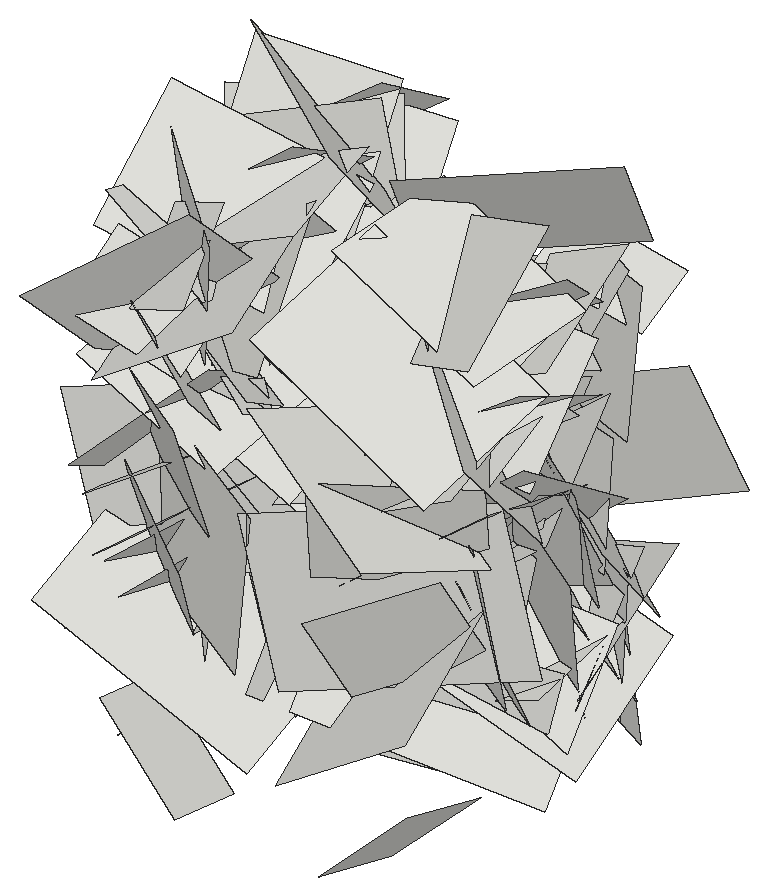
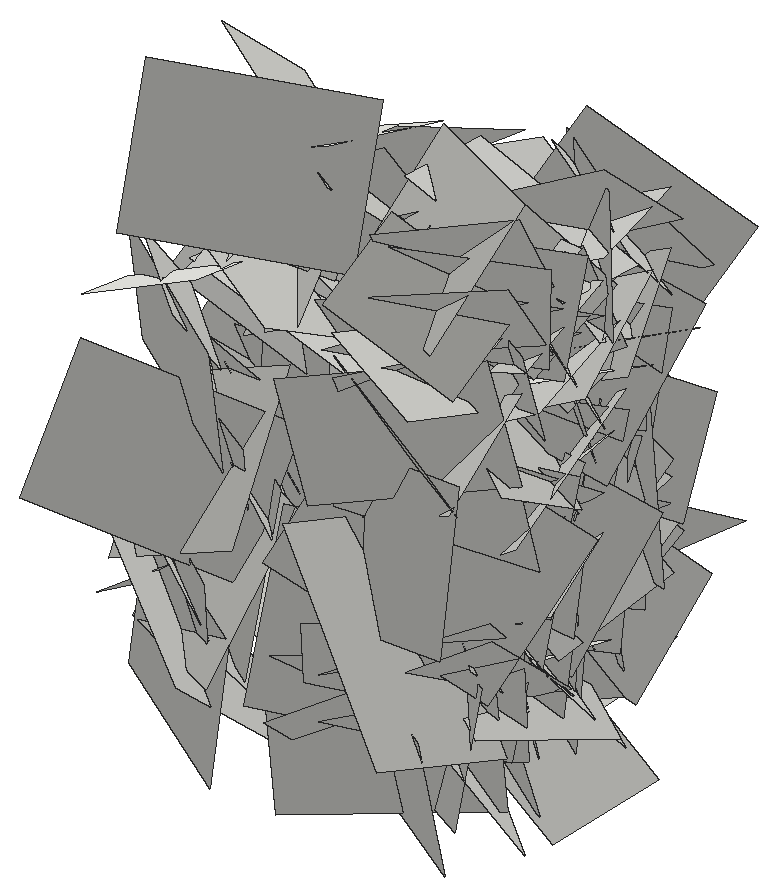
# SketchUp Ruby script. Lengths in inches.
U = 1.inch
M = Sketchup.active_model
def pt(a) = Geom::Point3d.new(a.map { |v| v * U })
def face(e, loops, mat)
  f = e.add_face(loops[0].map { |a| pt(a) })
  loops[1..].each { |l| e.add_face(l.map { |a| pt(a) }).erase! }
  f.material = f.back_material = mat if mat
  f
end
# faces: each face lists its corners as indices into pts; further lists are holes
def faces(e, pts, list, mat = nil) = list.each { |f| face(e, (f[0].is_a?(Array) ? f : [f]).map { |l| l.map { |i| pts[i] } }, mat) }
# xy, xz, yz: faces in a plane at the given z, y or x. An outline is a flat list of corners, or four numbers for a rectangle; further outlines are holes
def ring(l) = l.size == 4 ? [[l[0], l[1]], [l[2], l[1]], [l[2], l[3]], [l[0], l[3]]] : l.each_slice(2).to_a
def flat(e, list, mat, &to3) = list.each { |f| face(e, (f[0].is_a?(Array) ? f : [f]).map { |l| ring(l).map { |u, v| to3.(u, v) } }, mat) }
def xy(e, z, list, mat = nil) = flat(e, list, mat) { |x, y| [x, y, z] }
def xz(e, y, list, mat = nil) = flat(e, list, mat) { |x, z| [x, y, z] }
def yz(e, x, list, mat = nil) = flat(e, list, mat) { |y, z| [x, y, z] }
def lines(e, pts, list) = list.each { |a, b| e.add_line(pt(pts[a]), pt(pts[b])) }
# prism: a flat outline (further loops are holes) pulled along v
def prism(e, loops, v, mat = nil)
  f = face(e, loops, mat); d = Geom::Vector3d.new(v.map { |x| x * U })
  f.pushpull(f.normal.samedirection?(d) ? d.length : -d.length)
end
def box(e, o, s, mat = nil) = prism(e, [[o, [o[0] + s[0], o[1], o[2]], [o[0] + s[0], o[1] + s[1], o[2]], [o[0], o[1] + s[1], o[2]]]], [0, 0, s[2]], mat)
def at(x, y, z, deg = 0) = Geom::Transformation.translation(pt([x, y, z])) * Geom::Transformation.rotation(ORIGIN, Z_AXIS, deg.degrees)
def axes(o, x, y, z) = Geom::Transformation.new([*x, 0, *y, 0, *z, 0, *pt(o).to_a, 1])
def part(name) = M.definitions.add(name)
# library, detail: a bought-in or finely detailed component or shape, given as its bounding box
def library(name, o, s) = part(name).tap { |d| box(d.entities, o, s) }
def detail(e, o, s) = box(e.add_group.entities, o, s)
def put(e, d, t, mat = nil) = e.add_instance(d, t).tap { |i| i.material = mat if mat }
def group(e, t, mat = nil) = e.add_group.tap { |g| g.transformation = t; g.material = mat if mat }.entities
root = M.entities
c1 = part("Component\#6")
p = [[0.01,0,0],[0,3.24,4.54],[4.32,3.24,4.54],[4.33,0,0]]
faces(c1.entities,p,[[0,1,2,3]])
put(root,c1,axes([410.71,199.18,25.47],[0.11604,-0.3767,0.6399],[-0.02749,0.64448,0.38383],[0.78661,0.07809,-0.08099]))
put(root,c1,axes([410.71,201.02,32],[-0.03236,-0.79816,-0.43551],[-0.07074,-0.43262,0.79753],[0.9612,-0.0587,0.04403]))
put(root,c1,axes([414.68,202.06,39.63],[0.00244,-0.36914,-0.6705],[-0.07457,-0.66776,0.36739],[-0.80789,0.06052,-0.03594]))
put(root,c1,axes([410.71,194.18,31.13],[-0.04063,-0.16003,0.87853],[-0.02386,0.87924,0.15917],[0.94627,0.0153,0.04174]))
put(root,c1,axes([410.71,191.375,35.34],[0.1473,0.40574,0.51918],[0.07991,0.51733,-0.42447],[0.69387,-0.14571,-0.06134]))
put(root,c1,axes([414.68,192.92,34.17],[0.15147,-0.1521,1.01718],[0.1212,1.02293,0.1369],[-1.08344,0.09316,0.15752]))
put(root,c1,axes([414.68,201.02,39.48],[0.13577,0.09163,-0.9618],[0.05798,-0.96935,-0.08506],[-1.02248,-0.0428,-0.13253]))
put(root,c1,axes([414.68,193.07,33.95],[-0.05953,0.85388,-0.40475],[0.24794,-0.38029,-0.83472],[-0.97048,-0.14953,-0.18843]))
put(root,c1,axes([410.71,198.86,35.2],[-0.14047,0.16017,0.87964],[0.13868,0.88315,-0.1411],[0.93754,-0.10664,0.15267]))
put(root,c1,axes([410.71,198.41,25.5],[-0.14641,-1.02966,0.26735],[-0.10928,0.28128,1.03005],[1.12233,-0.10694,0.13517]))
put(root,c1,axes([414.68,192.38,31.46],[-0.05244,0.73173,-0.11131],[-0.01157,-0.11227,-0.73318],[-0.78447,-0.04726,0.01825]))
put(root,c1,axes([414.68,195.89,35.57],[0.03273,-0.74668,0.19464],[-0.06894,0.19158,0.74527],[-0.81502,-0.04619,-0.05522]))
put(root,c1,axes([410.71,195.33,34.42],[0.12228,0.30682,0.85432],[-0.19875,0.85067,-0.2802],[0.94146,0.13973,-0.17012]))
put(root,c1,axes([410.71,197.53,26.62],[0.11622,-0.11144,-0.6986],[0.08861,-0.69994,0.12478],[0.74462,0.10068,0.09418]))
put(root,c1,axes([414.68,194.17,31.15],[0.1572,-0.65225,0.62778],[0.00257,0.63643,0.66066],[-0.9596,-0.10514,0.10461]))
put(root,c1,axes([414.68,196.95,39.61],[0.06663,0.78722,-0.39485],[0.0883,-0.3994,-0.78302],[-0.92935,0.01849,-0.10271]))
put(root,c1,axes([410.71,195.16,37.28],[0.08536,-0.54597,-0.55526],[0.06407,-0.55215,0.55168],[0.82294,0.09962,0.01464]))
put(root,c1,axes([410.71,201.91,26.14],[-0.02369,0.31708,-0.9382],[-0.09459,-0.93526,-0.31396],[1.04548,-0.07743,-0.04967]))
put(root,c1,axes([414.68,198.57,33.25],[0.09717,0.14422,-0.89801],[0.11089,-0.89824,-0.13357],[-0.95769,-0.08937,-0.10658]))
put(root,c1,axes([410.71,200.1,34.99],[0.01875,0.74709,-0.59948],[-0.09315,-0.59579,-0.74508],[1.01106,-0.06874,-0.05753]))
put(root,c1,axes([414.68,192.15,39.48],[0.21361,0.71392,-0.72381],[0.12034,-0.74908,-0.70723],[-1.07091,0.05823,-0.22384]))
put(root,c1,axes([410.71,204.82,25.65],[-0.12938,-0.11687,-1.00907],[0.02351,-1.01639,0.11504],[1.07651,0.00815,-0.12379]))
put(root,c1,axes([414.68,197.17,21.41],[0.31691,0.51794,0.91951],[0.05422,0.94746,-0.55031],[-1.11735,0.19287,0.23409]))
put(root,c1,axes([410.71,195.4,26.27],[0.15303,-0.80886,0.21466],[-0.08059,0.20425,0.82078],[0.8834,0.15875,0.0377]))
put(root,c1,axes([410.71,195.7,29.31],[-0.12944,0.87645,-0.3909],[0.13192,-0.37627,-0.88251],[1.00866,0.16168,0.06525]))
put(root,c1,axes([414.68,199.74,34.07],[-0.11183,-0.60219,-0.2199],[0.02555,-0.22643,0.6085],[-0.67907,0.09065,0.0591]))
put(root,c1,axes([414.68,201.07,39.9375],[0.03161,0.68058,-0.41337],[0.06223,-0.41441,-0.67806],[-0.84176,-0.00508,-0.06565]))
put(root,c1,axes([410.71,195.45,23.05],[0.08121,0.42866,0.62692],[0.16296,0.6083,-0.43472],[0.78836,-0.1699,0.02528]))
put(root,c1,axes([414.68,196.5,26.6],[0.00001,0.64808,0.59207],[0.20568,0.57742,-0.63205],[-0.90746,0.13088,-0.14325]))
put(root,c1,axes([410.71,200.17,25.9],[0.12286,-0.34825,-0.84521],[-0.12526,-0.85054,0.33424],[0.96086,-0.06635,0.15165]))
put(root,c1,axes([410.71,194.92,22.54],[0.07164,-0.895,0.57486],[-0.24411,0.55005,0.88344],[1.1008,0.18023,0.15849]))
put(root,c1,axes([410.71,198.72,19.65],[-0.06387,-1.04135,0.05905],[-0.06023,0.06234,1.04135],[1.10396,-0.05685,0.06023]))
put(root,c1,axes([410.71,204.74,34.65],[0.08046,-0.48471,-0.63269],[0.12911,-0.62103,0.49039],[0.83492,0.14274,-0.01486]))
put(root,c1,axes([414.68,192.68,25.51],[-0.10584,0.56729,0.32604],[0.07365,0.33715,-0.56532],[-0.68964,-0.05105,-0.11041]))
put(root,c1,axes([410.71,194.12,36.42],[-0.16155,0.92195,-0.51802],[0.06641,-0.51458,-0.93426],[1.119,0.16364,-0.01934]))
put(root,c1,axes([414.68,197.11,20.7],[0.0234,0.20043,0.60552],[-0.11848,0.59772,-0.19378],[-0.66563,-0.09934,0.05578]))
put(root,c1,axes([410.71,192.76,27.5],[-0.21382,-0.08753,1.03604],[0.20559,1.03367,0.1251],[1.08277,-0.21355,0.18084]))
put(root,c1,axes([414.68,194.1,30.97],[0.07757,0.18705,0.69229],[-0.05179,0.69557,-0.18277],[-0.75837,-0.02837,0.08329]))
put(root,c1,axes([414.68,192.62,23.41],[0.0945,0.05137,0.75973],[-0.00531,0.76494,-0.05113],[-0.80713,0.00098,0.08928]))
put(root,c1,axes([414.68,194.0625,27.88],[0.03826,-0.32146,0.75655],[0.14724,0.74878,0.31153],[-0.85881,0.11405,0.08712]))
put(root,c1,axes([410.71,200.08,36.17],[0.04967,-0.3024,-0.77978],[0.15753,-0.76557,0.30582],[0.87244,0.15545,-0.01082]))
put(root,c1,axes([410.71,196.41,37.05],[0.02372,0.78814,-0.36288],[0.15491,-0.36124,-0.77556],[0.90659,0.0411,0.14202]))
put(root,c1,axes([410.71,206.72,25.52],[-0.07134,-1.27871,-0.42932],[-0.37284,-0.39835,1.24159],[1.38032,-0.17369,0.31318]))
put(root,c1,axes([410.71,198.67,35.61],[-0.10111,0.59855,0.78971],[0.15679,0.79307,-0.58323],[1.03859,-0.06146,0.16492]))
put(root,c1,axes([414.68,194.71,36.49],[0.01491,0.71707,-0.22931],[0.11795,-0.22881,-0.70868],[-0.78925,-0.02064,-0.11024]))
put(root,c1,axes([414.68,193.25,29.42],[0.0602,0.67546,-0.3863],[0.10598,-0.39045,-0.66802],[-0.81797,-0.00088,-0.11498]))
put(root,c1,axes([414.68,198.68,37.125],[-0.06347,0.58127,-0.24952],[0.07215,-0.24326,-0.58302],[-0.66662,-0.08167,-0.03935]))
put(root,c1,axes([410.71,195.125,35.61],[0.03117,0.92717,-0.40656],[-0.02653,-0.40594,-0.92757],[1.07281,-0.03698,-0.01113]))
put(root,c1,axes([414.68,200.57,36.04],[0.10099,0.61602,0.17436],[-0.1325,0.19079,-0.60575],[-0.66557,0.05549,0.14705]))
put(root,c1,axes([410.71,197.34,38.49],[0.22162,0.66132,-0.53694],[-0.02723,-0.54773,-0.68462],[0.90256,-0.17891,0.1112]))
put(root,c1,axes([410.71,198.8,27.02],[-0.0226,-0.2767,0.96977],[0.06915,0.96758,0.27751],[1.06674,-0.06859,0.00256]))
put(root,c1,axes([410.71,193.58,33.2],[0.1306,0.22319,-0.86205],[0.05382,-0.87061,-0.21815],[0.94237,0.01879,0.13193]))
put(root,c1,axes([410.71,197.85,24.73],[-0.35143,-0.52734,1.13432],[0.18025,1.14359,0.58135],[1.31365,-0.29799,0.22369]))
put(root,c1,axes([414.68,196.3,29.33],[0.09147,0.43894,-0.4809],[-0.05464,-0.47898,-0.44644],[-0.688,0.09639,-0.02848]))
put(root,c1,axes([414.68,192.39,25.48],[0.15082,-0.34829,0.66058],[0.01541,0.67363,0.35204],[-0.79143,-0.05326,0.13274]))
put(root,c1,axes([410.71,199.8,22.82],[-0.00598,0.07204,1.08492],[-0.02761,1.08461,-0.07215],[1.15221,0.02636,0.0039]))
put(root,c1,axes([414.68,194.26,19.42],[0.05867,-0.70774,0.13488],[0.12622,0.14241,0.69835],[-0.75321,-0.03127,0.12754]))
put(root,c1,axes([410.71,196.22,30.25],[-0.08073,-0.93811,0.99109],[-0.27356,0.98462,0.91216],[1.42044,0.13631,0.232]))
put(root,c1,axes([410.71,191.97,33.56],[0.08688,0.89449,0.25558],[0.12211,0.24484,-0.89383],[0.97851,-0.10998,0.08885]))
put(root,c1,axes([410.71,197.83,24.35],[-0.09568,0.96283,0.81475],[-0.1112,0.80827,-0.9668],[1.33234,0.1366,-0.02218]))
put(root,c1,axes([410.71,199.05,27.98],[0.08019,0.19915,0.92966],[0.13728,0.92174,-0.20799],[0.9984,-0.14274,-0.04607]))
put(root,c1,axes([410.71,202.95,33.21],[-0.17447,0.42234,-1.07867],[0.17991,-1.06896,-0.44444],[1.21466,0.21899,-0.08911]))
put(root,c1,axes([410.71,201.66,25.46],[-0.21728,-0.88431,0.94199],[0.03627,0.94972,0.89901],[1.36907,-0.16551,0.12568]))
put(root,c1,axes([410.71,195.04,27.27],[0.2131,0.57774,0.71728],[0.02179,0.73117,-0.59469],[0.97604,-0.14247,-0.14333]))
put(root,c1,axes([410.71,197.22,25.56],[0.17769,-0.12121,-0.94504],[0.07151,-0.95564,0.13453],[1.00742,0.08922,0.15714]))
put(root,c1,axes([410.71,192.77,37.47],[-0.01566,0.85002,0.74451],[0.07038,0.74394,-0.84805],[1.19569,-0.03266,0.05967]))
put(root,c1,axes([414.68,203.75,35.72],[0.12855,-0.35471,-0.52952],[0.05195,-0.53223,0.36775],[-0.67359,-0.10874,-0.07269]))
put(root,c1,axes([410.71,202.23,24.6],[-0.19755,-1.2824,-0.48224],[-0.04087,-0.48158,1.29554],[1.4517,-0.18807,-0.02915]))
put(root,c1,axes([410.71,200.11,31.93],[0.08158,0.26048,1.04137],[0.05734,1.04178,-0.26458],[1.13642,-0.07126,-0.06141]))
put(root,c1,axes([410.71,198.78,35.93],[0.06513,-0.64723,-0.92238],[0.00055,-0.92374,0.64822],[1.19442,0.03572,0.05]))
put(root,c1,axes([410.71,196.35,35.86],[0.06555,0.97369,0.5362],[0.0688,0.53295,-0.97527],[1.17625,-0.08544,0.02716]))
put(root,c1,axes([410.71,195.34,33.06],[0.01901,1.14103,-0.72029],[-0.19621,-0.71146,-1.13165],[1.41679,-0.11384,-0.14706]))
put(root,c1,axes([410.71,197.73,24.08],[0.06299,0.80841,0.87356],[-0.01823,0.87514,-0.8087],[1.26151,-0.02772,-0.0553]))
put(root,c1,axes([410.71,194.3,32.47],[-0.23408,0.14056,-1.33491],[0.22407,-1.33233,-0.17526],[1.40507,0.23589,-0.19445]))
put(root,c1,axes([410.71,196.04,25.17],[0.02819,1.07686,0.22249],[0.25409,0.21152,-1.05244],[1.13755,-0.07393,0.22957]))
put(root,c1,axes([410.71,193.85,32.27],[0.12737,1.17977,-0.33684],[-0.1012,-0.32843,-1.18439],[1.29659,-0.14153,-0.05935]))
put(root,c1,axes([410.71,198.24,37.08],[0.15669,-0.99926,-0.19378],[0.22295,-0.1616,0.99377],[1.05566,0.18244,-0.18112]))
put(root,c1,axes([410.71,197.21,31.46],[0.04455,0.58157,-0.95839],[0.2239,-0.94599,-0.56478],[1.16701,0.1593,0.14494]))
put(root,c1,axes([410.71,200.75,21.625],[0.14431,-0.01788,1.13958],[0.06693,1.14604,0.01044],[1.20625,-0.06145,-0.13692]))
put(root,c1,axes([410.71,198.29,23.22],[0.04433,-0.32511,1.32538],[-0.126,1.3201,0.32757],[1.44106,0.12543,-0.01213]))
put(root,c1,axes([410.71,196.35,30.1],[0.25467,1.00338,0.64071],[-0.12934,0.67094,-1.00496],[1.25528,-0.13443,-0.23354]))
put(root,c1,axes([410.71,199.72,26.12],[-0.08735,-0.8928,-1.02237],[0.07635,-1.02569,0.88989],[1.43674,0.00023,-0.10945]))
put(root,c1,axes([410.71,196.54,35.06],[0.17609,-1.11494,-0.45613],[-0.00034,-0.46049,1.12547],[1.27691,0.15363,0.0632]))
put(root,c1,axes([410.71,189.88,26.35],[0.12674,1.17916,0.69894],[-0.07675,0.70605,-1.17877],[1.45096,-0.06565,-0.1234]))
put(root,c1,axes([410.71,194.52,25.48],[0.11423,-0.20624,1.26777],[0.06819,1.2715,0.20138],[1.3598,-0.04643,-0.1166]))
put(root,c1,axes([410.71,199.97,41.09],[0.2759,0.65189,-0.94787],[0.07756,-0.97924,-0.65337],[1.21695,-0.08538,0.25653]))
put(root,c1,axes([410.71,200.57,23.13],[0.2198,-0.69796,1.13548],[-0.0671,1.14269,0.71395],[1.41122,0.16304,-0.1429]))
put(root,c1,axes([410.71,195.625,24.52],[0.22176,-0.47224,1.18941],[0.10161,1.2076,0.46259],[1.3527,-0.0133,-0.22974]))
put(root,c1,axes([410.71,193.54,33.12],[0.22081,1.30446,0.31828],[0.37279,0.25784,-1.28691],[1.3736,-0.27967,0.29809]))
put(root,c1,axes([424.49,193.54,33.12],[-0.22081,1.30446,0.31828],[-0.37279,0.25784,-1.28691],[-1.3736,-0.27967,0.29809]))
put(root,c1,axes([424.49,195.625,24.52],[-0.22176,-0.47224,1.18941],[-0.10161,1.2076,0.46259],[-1.3527,-0.0133,-0.22974]))
put(root,c1,axes([424.49,200.57,23.13],[-0.2198,-0.69796,1.13548],[0.0671,1.14269,0.71395],[-1.41122,0.16304,-0.1429]))
put(root,c1,axes([424.49,199.97,41.09],[-0.2759,0.65189,-0.94787],[-0.07756,-0.97924,-0.65337],[-1.21695,-0.08538,0.25653]))
put(root,c1,axes([424.49,193.84,30.46],[-0.25587,-1.06575,0.3461],[-0.15582,0.3811,1.07099],[-1.17751,0.18115,-0.21693]))
put(root,c1,axes([424.49,194.52,25.48],[-0.11423,-0.20624,1.26777],[-0.06819,1.2715,0.20138],[-1.3598,-0.04643,-0.1166]))
put(root,c1,axes([424.49,189.88,26.35],[-0.12674,1.17916,0.69894],[0.07675,0.70605,-1.17877],[-1.45096,-0.06565,-0.1234]))
put(root,c1,axes([424.49,196.54,35.06],[-0.17609,-1.11494,-0.45613],[0.00034,-0.46049,1.12547],[-1.27691,0.15363,0.0632]))
put(root,c1,axes([424.49,199.72,26.12],[0.08735,-0.8928,-1.02237],[-0.07635,-1.02569,0.88989],[-1.43674,0.00023,-0.10945]))
put(root,c1,axes([424.49,196.35,30.1],[-0.25467,1.00338,0.64071],[0.12934,0.67094,-1.00496],[-1.25528,-0.13443,-0.23354]))
put(root,c1,axes([424.49,198.29,23.22],[-0.04433,-0.32511,1.32538],[0.126,1.3201,0.32757],[-1.44106,0.12543,-0.01213]))
put(root,c1,axes([424.49,200.75,21.625],[-0.14431,-0.01788,1.13958],[-0.06693,1.14604,0.01044],[-1.20625,-0.06145,-0.13692]))
put(root,c1,axes([424.49,197.21,31.46],[-0.04455,0.58157,-0.95839],[-0.2239,-0.94599,-0.56478],[-1.16701,0.1593,0.14494]))
put(root,c1,axes([424.49,198.24,37.08],[-0.15669,-0.99926,-0.19378],[-0.22295,-0.1616,0.99377],[-1.05566,0.18244,-0.18112]))
put(root,c1,axes([424.49,193.85,32.27],[-0.12737,1.17977,-0.33684],[0.1012,-0.32843,-1.18439],[-1.29659,-0.14153,-0.05935]))
put(root,c1,axes([424.49,196.04,25.17],[-0.02819,1.07686,0.22249],[-0.25409,0.21152,-1.05244],[-1.13755,-0.07393,0.22957]))
put(root,c1,axes([424.49,194.3,32.47],[0.23408,0.14056,-1.33491],[-0.22407,-1.33233,-0.17526],[-1.40507,0.23589,-0.19445]))
put(root,c1,axes([424.49,197.73,24.08],[-0.06299,0.80841,0.87356],[0.01823,0.87514,-0.8087],[-1.26151,-0.02772,-0.0553]))
put(root,c1,axes([424.49,195.34,33.06],[-0.01901,1.14103,-0.72029],[0.19621,-0.71146,-1.13165],[-1.41679,-0.11384,-0.14706]))
put(root,c1,axes([424.49,196.35,35.86],[-0.06555,0.97369,0.5362],[-0.0688,0.53295,-0.97527],[-1.17625,-0.08544,0.02716]))
put(root,c1,axes([424.49,198.78,35.93],[-0.06513,-0.64723,-0.92238],[-0.00055,-0.92374,0.64822],[-1.19442,0.03572,0.05]))
put(root,c1,axes([424.49,200.11,31.93],[-0.08158,0.26048,1.04137],[-0.05734,1.04178,-0.26458],[-1.13642,-0.07126,-0.06141]))
put(root,c1,axes([424.49,202.23,24.6],[0.19755,-1.2824,-0.48224],[0.04087,-0.48158,1.29554],[-1.4517,-0.18807,-0.02915]))
put(root,c1,axes([420.52,203.75,35.72],[-0.12855,-0.35471,-0.52952],[-0.05195,-0.53223,0.36775],[0.67359,-0.10874,-0.07269]))
put(root,c1,axes([424.49,192.77,37.47],[0.01566,0.85002,0.74451],[-0.07038,0.74394,-0.84805],[-1.19569,-0.03266,0.05967]))
put(root,c1,axes([424.49,197.22,25.56],[-0.17769,-0.12121,-0.94504],[-0.07151,-0.95564,0.13453],[-1.00742,0.08922,0.15714]))
put(root,c1,axes([424.49,195.04,27.27],[-0.2131,0.57774,0.71728],[-0.02179,0.73117,-0.59469],[-0.97604,-0.14247,-0.14333]))
put(root,c1,axes([424.49,201.66,25.46],[0.21728,-0.88431,0.94199],[-0.03627,0.94972,0.89901],[-1.36907,-0.16551,0.12568]))
put(root,c1,axes([424.49,202.95,33.21],[0.17447,0.42234,-1.07867],[-0.17991,-1.06896,-0.44444],[-1.21466,0.21899,-0.08911]))
put(root,c1,axes([424.49,199.05,27.98],[-0.08019,0.19915,0.92966],[-0.13728,0.92174,-0.20799],[-0.9984,-0.14274,-0.04607]))
put(root,c1,axes([424.49,197.83,24.35],[0.09568,0.96283,0.81475],[0.1112,0.80827,-0.9668],[-1.33234,0.1366,-0.02218]))
put(root,c1,axes([424.49,191.97,33.56],[-0.08688,0.89449,0.25558],[-0.12211,0.24484,-0.89383],[-0.97851,-0.10998,0.08885]))
put(root,c1,axes([424.49,196.22,30.25],[0.08073,-0.93811,0.99109],[0.27356,0.98462,0.91216],[-1.42044,0.13631,0.232]))
put(root,c1,axes([420.52,194.26,19.42],[-0.05867,-0.70774,0.13488],[-0.12622,0.14241,0.69835],[0.75321,-0.03127,0.12754]))
put(root,c1,axes([424.49,199.8,22.82],[0.00598,0.07204,1.08492],[0.02761,1.08461,-0.07215],[-1.15221,0.02636,0.0039]))
put(root,c1,axes([420.52,192.39,25.48],[-0.15082,-0.34829,0.66058],[-0.01541,0.67363,0.35204],[0.79143,-0.05326,0.13274]))
put(root,c1,axes([420.52,196.3,29.33],[-0.09147,0.43894,-0.4809],[0.05464,-0.47898,-0.44644],[0.688,0.09639,-0.02848]))
put(root,c1,axes([424.49,197.85,24.73],[0.35143,-0.52734,1.13432],[-0.18025,1.14359,0.58135],[-1.31365,-0.29799,0.22369]))
put(root,c1,axes([424.49,193.58,33.2],[-0.1306,0.22319,-0.86205],[-0.05382,-0.87061,-0.21815],[-0.94237,0.01879,0.13193]))
put(root,c1,axes([424.49,198.8,27.02],[0.0226,-0.2767,0.96977],[-0.06915,0.96758,0.27751],[-1.06674,-0.06859,0.00256]))
put(root,c1,axes([424.49,197.34,38.49],[-0.22162,0.66132,-0.53694],[0.02723,-0.54773,-0.68462],[-0.90256,-0.17891,0.1112]))
put(root,c1,axes([420.52,200.57,36.04],[-0.10099,0.61602,0.17436],[0.1325,0.19079,-0.60575],[0.66557,0.05549,0.14705]))
put(root,c1,axes([424.49,195.125,35.61],[-0.03117,0.92717,-0.40656],[0.02653,-0.40594,-0.92757],[-1.07281,-0.03698,-0.01113]))
put(root,c1,axes([420.52,198.68,37.125],[0.06347,0.58127,-0.24952],[-0.07215,-0.24326,-0.58302],[0.66662,-0.08167,-0.03935]))
